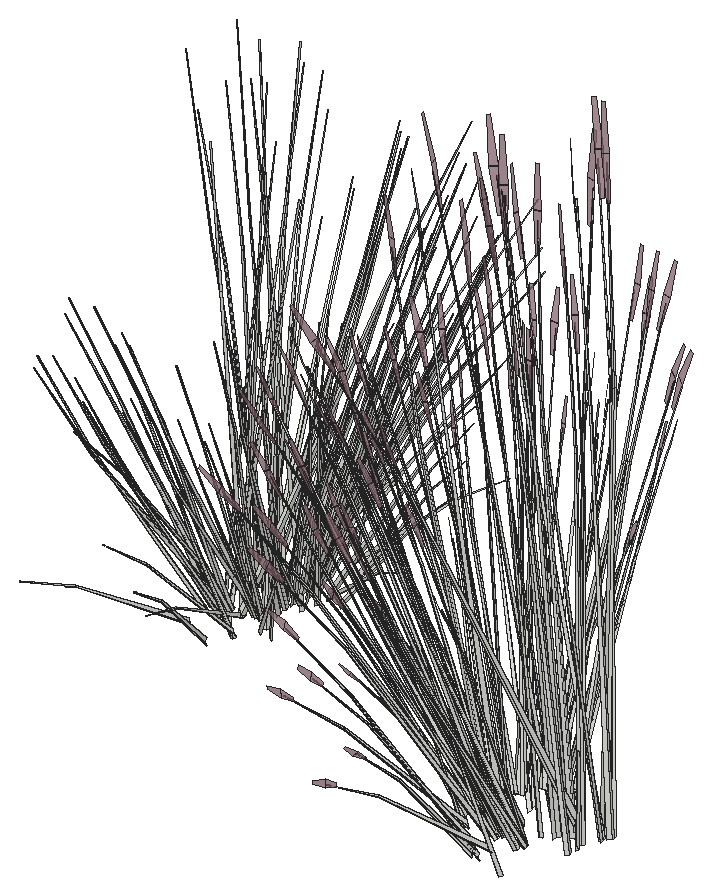
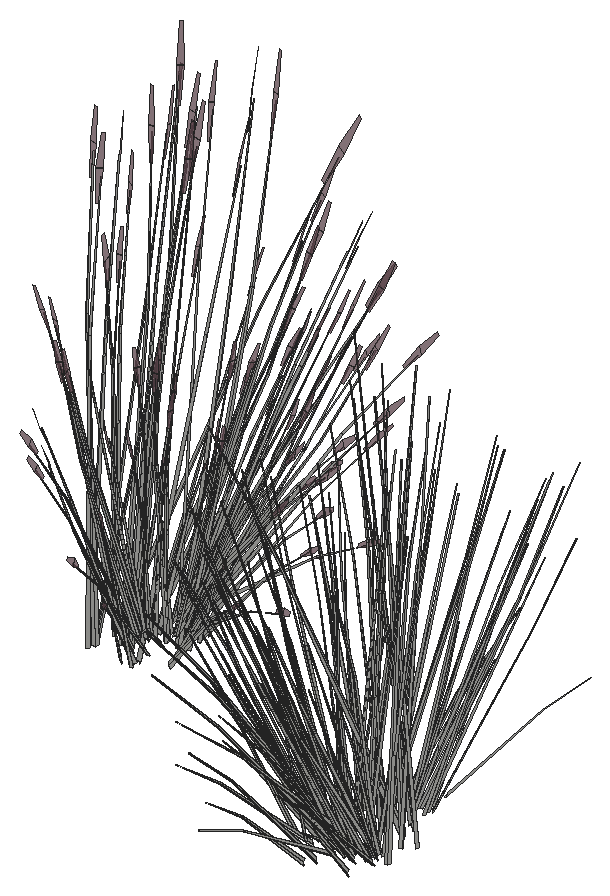
# SketchUp Ruby script. Lengths in inches.
U = 1.inch
M = Sketchup.active_model
def pt(a) = Geom::Point3d.new(a.map { |v| v * U })
def face(e, loops, mat)
  f = e.add_face(loops[0].map { |a| pt(a) })
  loops[1..].each { |l| e.add_face(l.map { |a| pt(a) }).erase! }
  f.material = f.back_material = mat if mat
  f
end
# faces: each face lists its corners as indices into pts; further lists are holes
def faces(e, pts, list, mat = nil) = list.each { |f| face(e, (f[0].is_a?(Array) ? f : [f]).map { |l| l.map { |i| pts[i] } }, mat) }
# xy, xz, yz: faces in a plane at the given z, y or x. An outline is a flat list of corners, or four numbers for a rectangle; further outlines are holes
def ring(l) = l.size == 4 ? [[l[0], l[1]], [l[2], l[1]], [l[2], l[3]], [l[0], l[3]]] : l.each_slice(2).to_a
def flat(e, list, mat, &to3) = list.each { |f| face(e, (f[0].is_a?(Array) ? f : [f]).map { |l| ring(l).map { |u, v| to3.(u, v) } }, mat) }
def xy(e, z, list, mat = nil) = flat(e, list, mat) { |x, y| [x, y, z] }
def xz(e, y, list, mat = nil) = flat(e, list, mat) { |x, z| [x, y, z] }
def yz(e, x, list, mat = nil) = flat(e, list, mat) { |y, z| [x, y, z] }
def lines(e, pts, list) = list.each { |a, b| e.add_line(pt(pts[a]), pt(pts[b])) }
# prism: a flat outline (further loops are holes) pulled along v
def prism(e, loops, v, mat = nil)
  f = face(e, loops, mat); d = Geom::Vector3d.new(v.map { |x| x * U })
  f.pushpull(f.normal.samedirection?(d) ? d.length : -d.length)
end
def box(e, o, s, mat = nil) = prism(e, [[o, [o[0] + s[0], o[1], o[2]], [o[0] + s[0], o[1] + s[1], o[2]], [o[0], o[1] + s[1], o[2]]]], [0, 0, s[2]], mat)
def at(x, y, z, deg = 0) = Geom::Transformation.translation(pt([x, y, z])) * Geom::Transformation.rotation(ORIGIN, Z_AXIS, deg.degrees)
def axes(o, x, y, z) = Geom::Transformation.new([*x, 0, *y, 0, *z, 0, *pt(o).to_a, 1])
def part(name) = M.definitions.add(name)
# library, detail: a bought-in or finely detailed component or shape, given as its bounding box
def library(name, o, s) = part(name).tap { |d| box(d.entities, o, s) }
def detail(e, o, s) = box(e.add_group.entities, o, s)
def put(e, d, t, mat = nil) = e.add_instance(d, t).tap { |i| i.material = mat if mat }
def group(e, t, mat = nil) = e.add_group.tap { |g| g.transformation = t; g.material = mat if mat }.entities
root = M.entities
M.materials.add("LightPink_Translucent").color = [144, 107, 117]
M.materials["LightPink_Translucent"].alpha = 0.75
c1 = part("blade")
p = [[2.15,0.21,22],[0,0.17,0],[0.09,0.45,0],[2.18,0.31,22],[2.29,0.31,22],[0.38,0.45,0],
  [2.48,0.24,33],[2.49,0.24,33],[2.48,0.22,33]]
faces(c1.entities,p,[[0,1,2,3],[4,5,2,3],[6,3,4,7],[8,0,3,6]])
c2 = part("blade with seeds\#1")
put(c2.entities,c1,at(0,0,0))
c3 = part("seeds")
p = [[0.3,-0.1,1.38],[-0.01,-0.03,1.59],[-0.01,-0.03,0.03],[0.14,-0.07,-0.07],[0.29,-0.03,3],[0.15,0.01,3.11]]
faces(c3.entities,p,[[0,1,2,3],[1,0,4,5]],"LightPink_Translucent")
c4 = part("blade with seeds")
put(c4.entities,c1,at(0,0,0))
put(c4.entities,c3,axes([2.4,0.25,30.99],[1.5799,-0.05474,1.17369],[-0.12525,1.92788,0.29478],[-0.07173,-0.02425,1.56792]))
put(root,c2,axes([216.32,38.09,16.14],[-0.56782,-0.84974,0.42031],[0.60301,-0.73285,0.34656],[-0.10474,0.39867,0.86972]))
put(root,c2,axes([220.11,33.5,14.76],[0.31026,-0.88918,1.18253],[0.6684,0.87109,0.46763],[-0.39615,0.39018,0.99135]))
put(root,c2,axes([216.32,37.7,15.86],[-0.58508,-0.05181,0.05027],[0.01604,-0.78236,0.39574],[-0.06122,0.29969,0.60345]))
put(root,c2,axes([216.5,38,15.7],[-0.48173,0.58546,-0.27686],[-0.45602,-0.6685,0.35743],[-0.06938,0.33965,0.68391]))
put(root,c2,axes([217.37,29.3,15.7],[-0.10996,-0.89566,-0.27686],[0.6286,-0.2365,0.35743],[-0.16884,-0.25667,0.68391]))
put(root,c2,axes([217.74,30.03,16.11],[0.10996,0.89566,0.27686],[-0.6286,0.2365,-0.35743],[-0.16884,-0.25667,0.68391]))
put(root,c2,axes([216.83,37.38,16.06],[-0.01853,1.02857,-0.55542],[-0.78011,-0.06908,0.06703],[-0.08233,0.43575,0.78569]))
put(root,c2,axes([217.5,29.41,15.86],[0.70813,-0.25519,0.37528],[0.1229,1.00103,0.30943],[-0.16654,-0.29502,0.77654]))
put(root,c2,axes([217.64,29.22,15.86],[0.32359,-0.70638,0.05027],[0.4608,0.41126,0.39574],[-0.14898,-0.22647,0.60345]))
put(root,c2,axes([218.36,26.72,15.85],[-0.1172,-0.14278,1.36768],[-0.7189,0.18276,-0.2163],[-0.1363,-0.35826,0.10969]))
put(root,c2,axes([215.55,38.78,15.84],[0.07678,-0.07628,1.38675],[0.69023,0.36774,-0.13103],[0.00499,0.37243,0.24541]))
put(root,c2,axes([216.98,37.73,15.82],[0.50967,0.74714,-0.39948],[-0.5384,0.65433,-0.30943],[-0.07755,0.37961,0.76437]))
put(root,c2,axes([216.76,37.17,16.11],[0.48173,-0.58546,0.27686],[0.45602,0.6685,-0.35743],[-0.06938,0.33965,0.68391]))
put(root,c2,axes([218.625,34.39,14.0625],[0.37292,-1.15935,0.18813],[0.77487,0.55796,0.39091],[-0.17862,0,1.25509]))
put(root,c2,axes([216.45,37.33,16.1],[0.78248,0.05509,-0.09507],[-0.02139,1.04315,-0.52766],[-0.05435,0.40176,0.80177]))
put(root,c2,axes([217.66,39.41,14.32],[-0.05506,-0.65692,0.89796],[0.4851,0.4167,0.65976],[-0.07277,0.32462,0.19778]))
put(root,c2,axes([218.11,34.77,14.29],[0.0475,1.11735,0.34976],[-0.78843,0.10105,-0.16833],[-0.07991,-0.20003,1.12298]))
put(root,c2,axes([219.45,29.53,16.1],[-0.69671,0.51771,-0.09507],[-0.34238,-0.91885,-0.52766],[-0.09192,-0.38721,0.80177]))
put(root,c2,axes([217.53,38.66,15.19],[-0.01743,-0.42679,1.33979],[0.75527,0.28313,0.10833],[-0.04672,0.60821,0.57275]))
put(root,c2,axes([218.85,29.57,15.82],[-0.69988,-0.27875,-0.39948],[0.23989,-0.95572,-0.30943],[-0.06417,-0.38479,0.76437]))
put(root,c2,axes([219.07,35.03,14.29],[0.6933,0.49923,0.34976],[-0.33366,1.03732,-0.16833],[-0.15982,0,1.12298]))
put(root,c2,axes([216.75,35.29,14.1],[0.76467,0.29724,0.13792],[-0.21639,1.08771,0.2743],[-0.00372,-0.1879,1.25403]))
put(root,c2,axes([219.11,29.75,16.06],[-0.33981,-0.90415,-0.55542],[0.69949,-0.50388,0.06703],[-0.07946,-0.43686,0.78569]))
put(root,c2,axes([219.24,29.89,16.11],[-0.21464,0.85512,0.27686],[-0.6262,-0.24941,-0.35743],[-0.05742,-0.34428,0.68391]))
put(root,c2,axes([218.1,38.84,15.86],[-0.70155,-0.2907,0.37528],[0.23989,-0.95572,0.30943],[0.04216,0.37584,0.77654]))
put(root,c2,axes([217.91,38.91,15.86],[-0.52462,0.37791,0.05027],[-0.25678,-0.68914,0.39574],[0.05066,0.30378,0.60345]))
put(root,c2,axes([217.78,33.43,14.29],[-0.64581,0.61812,0.34976],[-0.45477,-0.93627,-0.16833],[0.07991,-0.20003,1.12298]))
put(root,c2,axes([216.8,32,14.1],[0.20421,1.10567,0.13792],[-0.75999,0.27302,0.2743],[0.11073,-0.09861,1.25403]))
put(root,c2,axes([218.18,39.04,15.7],[-0.21464,0.85512,-0.27686],[-0.6262,-0.24941,0.35743],[0.05742,0.34428,0.68391]))
put(root,c2,axes([219.17,28.99,15.7],[0.21464,-0.85512,-0.27686],[0.6262,0.24941,0.35743],[-0.05742,-0.34428,0.68391]))
put(root,c2,axes([220.7,35.39,14.1],[-0.20421,-1.10567,0.13792],[0.75999,-0.27302,0.2743],[-0.11073,0.09861,1.25403]))
put(root,c2,axes([218.4,31.32,15.19],[0.01743,0.42679,1.33979],[-0.75527,-0.28313,0.10833],[0.04672,-0.60821,0.57275]))
put(root,c2,axes([219.4375,29.11,15.86],[0.52462,-0.37791,0.05027],[0.25678,0.68914,0.39574],[-0.05066,-0.30378,0.60345]))
put(root,c2,axes([219.25,29.18,15.86],[0.70155,0.2907,0.37528],[-0.23989,0.95572,0.30943],[-0.04216,-0.37584,0.77654]))
put(root,c2,axes([218.11,38.14,16.11],[0.21464,-0.85512,0.27686],[0.6262,0.24941,-0.35743],[0.05742,0.34428,0.68391]))
put(root,c2,axes([218.79,30.41,14.1],[-0.56045,0.80843,0.13792],[-0.5436,-0.81469,0.2743],[0.11446,0.08929,1.25403]))
put(root,c2,axes([218.07,36.43,14.77],[-0.1113,-0.29248,1.38425],[0.77713,-0.10086,0.10833],[0.10312,0.63351,0.49474]))
put(root,c2,axes([219.3,27.17,14.32],[0.12702,0.63574,0.89796],[-0.52496,-0.29925,0.65976],[0.03592,-0.33726,0.19778]))
put(root,c2,axes([220.74,32.1,14.1],[-0.76467,-0.29724,0.13792],[0.21639,-1.08771,0.2743],[0.00372,0.1879,1.25403]))
put(root,c2,axes([218.42,32.36,14.29],[-0.6933,-0.49923,0.34976],[0.33366,-1.03732,-0.16833],[0.15982,0,1.12298]))
put(root,c2,axes([218.5,38.45,15.82],[0.69988,0.27875,-0.39948],[-0.23989,0.95572,-0.30943],[0.06417,0.38479,0.76437]))
put(root,c2,axes([217.9,38.5,16.1],[0.69671,-0.51771,-0.09507],[0.34238,0.91885,-0.52766],[0.09192,0.38721,0.80177]))
put(root,c2,axes([221.52,27.47,15.84],[-0.06736,0.09304,1.38675],[-0.72203,-0.20352,-0.13103],[-0.04613,-0.36649,0.24541]))
put(root,c2,axes([218.59,39.58,15.85],[0.0999,0.16803,1.36768],[0.72987,-0.01429,-0.2163],[0.09492,0.38514,0.10969]))
put(root,c2,axes([220.92,28.28,15.23],[-0.64678,0.19693,-0.0273],[-0.14869,-0.93082,-0.12377],[0.041,-0.19438,0.40823]))
put(root,c2,axes([220.9,30.6875,16.1],[-0.78248,-0.05509,-0.09507],[0.02139,-1.04315,-0.52766],[0.05435,-0.40176,0.80177]))
put(root,c2,axes([219.39,32.625,14.29],[-0.0475,-1.11735,0.34976],[0.78843,-0.10105,-0.16833],[0.07991,0.20003,1.12298]))
put(root,c2,axes([220.59,30.85,16.11],[-0.48173,0.58546,0.27686],[-0.45602,-0.6685,-0.35743],[0.06938,-0.33965,0.68391]))
put(root,c2,axes([220.43,29.78,15.85],[-0.01301,-0.22073,1.36768],[-0.59776,-0.60543,-0.2163],[0.0789,-0.39262,0.10969]))
put(root,c2,axes([219.71,38.81,15.86],[-0.32359,0.70638,0.05027],[-0.4608,-0.41126,0.39574],[0.14898,0.22647,0.60345]))
put(root,c2,axes([219.85,38.61,15.86],[-0.70813,0.25519,0.37528],[-0.1229,-1.00103,0.30943],[0.16654,0.29502,0.77654]))
put(root,c2,axes([218.86,38.48,15.19],[-0.16275,-0.35702,1.33979],[0.75203,-0.30057,0.10833],[0.16997,0.56048,0.57275]))
put(root,c2,axes([220.52,30.64,16.06],[0.01853,-1.02857,-0.55542],[0.78011,0.06908,0.06703],[0.08233,-0.43575,0.78569]))
put(root,c2,axes([219.61,37.99,16.11],[-0.10996,-0.89566,0.27686],[0.6286,-0.2365,-0.35743],[0.16884,0.25667,0.68391]))
put(root,c2,axes([219.33,41.44,15.84],[0.02064,-0.13132,1.38675],[0.67982,-0.40623,-0.13103],[0.17843,0.26881,0.24541]))
put(root,c2,axes([219.98,38.72,15.7],[0.10996,0.89566,-0.27686],[-0.6286,0.2365,0.35743],[0.16884,0.25667,0.68391]))
put(root,c2,axes([220.85,30.02,15.7],[0.48173,-0.58546,-0.27686],[0.45602,0.6685,0.35743],[0.06938,-0.33965,0.68391]))
put(root,c2,axes([221.03,30.32,15.86],[0.58508,0.05181,0.05027],[-0.01604,0.78236,0.39574],[0.06122,-0.29969,0.60345]))
put(root,c2,axes([220.84,30.25,15.86],[0.50698,0.7587,0.37528],[-0.5384,0.65433,0.30943],[0.09352,-0.35595,0.77654]))
put(root,c2,axes([221.49,40.34,14.32],[-0.34872,-0.42882,0.89796],[0.55204,-0.16921,0.65976],[0.09885,0.30989,0.19778]))
put(root,c2,axes([217.87,32.05,15.66],[-0.39977,0.88912,1.08107],[-0.62243,-0.93883,0.46645],[0.3751,-0.28686,1.04495]))
put(root,c2,axes([219.61,32.12,15.19],[-0.13256,0.3822,1.33979],[-0.55613,-0.79096,0.10833],[0.25088,-0.49297,0.57275]))
put(root,c2,axes([221.39,40.03,16.58],[0.20538,-0.90798,-0.05072],[0.63212,0.2793,-0.22997],[0.09598,0.14851,0.75852]))
put(root,c2,axes([221.43,32.66,16.11],[-0.61974,0.15892,0.27686],[-0.16365,-0.90846,-0.35743],[0.1776,-0.24401,0.68391]))
put(root,c2,axes([219.55,38.46,16.1],[0.42425,-0.9518,-0.09507],[0.6144,0.54834,-0.52766],[0.21357,0.26891,0.80177]))
put(root,c2,axes([221.12,30.71,14.32],[-0.22123,0.57934,0.89796],[-0.22479,-0.74807,0.65976],[0.19041,-0.20177,0.19778]))
put(root,c2,axes([219.36,37.18,15.19],[-0.23641,-0.257,1.33979],[0.63812,-0.64891,0.10833],[0.2906,0.44508,0.57275]))
put(root,c2,axes([220.05,37.99,15.82],[0.70255,-0.26433,-0.39948],[0.1229,1.00103,-0.30943],[0.1887,0.28686,0.76437]))
put(root,c2,axes([221.75,32.74,16.1],[-0.65859,-0.61314,-0.09507],[0.37942,-0.88794,-0.52766],[0.18607,-0.30866,0.80177]))
put(root,c2,axes([218.63,32.12,14.38],[-0.72443,0.02811,1.10444],[0.18779,-1.27212,0.46763],[0.3964,0.30088,1.0425]))
put(root,c2,axes([220.86,36.78,16.11],[-0.4051,-0.6962,0.27686],[0.46256,-0.65905,-0.35743],[0.23502,0.10028,0.68391]))
put(root,c2,axes([221.23,37.42,15.86],[-0.03585,0.84557,0.05027],[-0.54135,-0.02318,0.39574],[0.20737,0.08848,0.60345]))
put(root,c2,axes([222.3,33.55,15.84],[-0.09315,-0.00304,1.38675],[-0.41098,-0.88177,-0.13103],[0.14669,-0.30629,0.24541]))
put(root,c2,axes([221.28,37.15,15.86],[-0.52497,0.7327,0.37528],[-0.45276,-0.77811,0.30943],[0.2463,0.13515,0.77654]))
put(root,c2,axes([221.42,32.02,15.82],[-0.1829,-1.01534,-0.39948],[0.69265,-0.17761,-0.30943],[0.19849,-0.27272,0.76437]))
put(root,c2,axes([221.53,34.83,16.11],[-0.59169,-0.3102,0.27686],[0.17258,-0.905,-0.35743],[0.23822,-0.08298,0.68391]))
put(root,c2,axes([222.125,30.62,14.25],[-0.02413,0.65983,0.82134],[-0.51251,-0.43575,0.45348],[0.18208,-0.26066,0.64427]))
put(root,c2,axes([221.99,32.52,15.86],[0.48877,0.46765,0.05027],[-0.28456,0.66596,0.39574],[0.1567,-0.2153,0.60345]))
put(root,c2,axes([221.86,32.32,15.86],[0.17657,1.0234,0.37528],[-0.69265,0.17761,0.30943],[0.20414,-0.24069,0.77654]))
put(root,c2,axes([219.95,37.37,15.19],[-0.26446,-0.19158,1.33979],[0.54729,-0.80372,0.10833],[0.3411,0.36257,0.57275]))
put(root,c2,axes([223.64,33.61,16.58],[-0.4414,-0.71104,-0.05072],[0.48343,-0.65151,-0.22997],[0.13698,-0.04587,0.75852]))
put(root,c2,axes([221.4375,37.15,15.7],[0.4051,0.6962,-0.27686],[-0.46256,0.65905,0.35743],[0.23502,0.10028,0.68391]))
put(root,c2,axes([222.06,35.11,15.86],[0.26149,0.75819,0.05027],[-0.47684,0.37111,0.39574],[0.2102,-0.07322,0.60345]))
put(root,c2,axes([221.32,39.55,15.85],[0.15226,0.02558,1.36768],[0.52969,-0.72584,-0.2163],[0.25048,0.19002,0.10969]))
put(root,c2,axes([220.97,37.23,16.38],[0.03812,-1.13085,-0.10552],[0.7218,0.03091,-0.5857],[0.27799,0.07855,0.88996]))
put(root,c2,axes([222.01,34.84,16.12],[-0.20115,1.01389,0.41656],[-0.6613,-0.3467,0.34347],[0.26006,-0.06093,0.86196]))
put(root,c2,axes([221.78,35.14,16.1],[-0.35822,-1.00689,-0.09507],[0.63579,-0.49481,-0.52766],[0.26792,-0.13285,0.80177]))
put(root,c2,axes([223.01,36.7,14.32],[-0.4575,0.02663,0.89796],[0.32631,-0.6654,0.65976],[0.21806,0.13086,0.19778]))
put(root,c2,axes([221.25,36.46,16.07],[0.51698,-0.73658,-0.44342],[0.45276,0.77811,-0.34347],[0.26267,0.11207,0.84845]))
put(root,c2,axes([220.38,33.7,15.19],[-0.24703,0.23521,1.33979],[-0.20797,-1.08685,0.10833],[0.38782,-0.24564,0.57275]))
put(root,c2,axes([221.75,34.27,15.82],[0.19288,-1.01147,-0.39948],[0.6613,0.3467,-0.30943],[0.26625,-0.09275,0.76437]))
put(root,c2,axes([222.15,34.73,15.7],[0.59169,0.3102,-0.27686],[-0.17258,0.905,0.35743],[0.23822,-0.08298,0.68391]))
put(root,c2,axes([221.01,36.68,16.33],[0.71171,0.02677,-0.61651],[-0.0478,1.12742,0.0744],[0.30151,0.11898,0.87212]))
put(root,c2,axes([220.5,35.62,15.19],[-0.29531,0.02518,1.33979],[0.19591,-1.09152,0.10833],[0.42084,0.06751,0.57275]))
put(root,c2,axes([222.88,39.63,15.84],[-0.04645,-0.11673,1.38675],[0.30899,-0.96483,-0.13103],[0.25727,0.02267,0.24541]))
put(root,c2,axes([221.62,34.64,16.06],[0.62562,-0.4911,-0.55542],[0.34866,1.01092,0.06703],[0.30228,-0.11484,0.78569]))
put(root,c2,axes([223.2,35.375,15.85],[0.1239,-0.13043,1.36768],[0.04868,-1.05257,-0.2163],[0.27325,-0.10585,0.10969]))
put(root,c2,axes([222.01,37.0625,14.79],[-0.3972,-0.02261,1.20664],[0.2098,-1.0168,0.16675],[0.42332,0.0881,0.56978]))
put(root,c4,axes([250.125,18.36,15.95],[0.4003,-0.02088,1.4862],[-0.26555,0.90478,0.12017],[-0.57046,-0.05596,0.63534]))
put(root,c4,axes([250.29,19.95,15.95],[0.33486,-0.19497,1.4862],[0.28191,0.90091,0.12017],[-0.52569,0.20361,0.63534]))
put(root,c4,axes([249.25,21.49,14.84],[0.33539,0.07567,1.24013],[0.21617,0.77287,-0.2667],[-0.45558,0.14467,0.53022]))
put(root,c4,axes([252.22,19.01,15.49],[0.27432,-0.13334,1.53553],[0.0946,0.93098,0.12017],[-0.59418,0.12354,0.54881]))
put(root,c4,axes([249.27,19.64,16.68],[-0.1576,0.11967,1.51715],[0.01341,0.87436,-0.23994],[-0.36123,0.11371,0.12168]))
put(root,c4,axes([251.32,17.52,16.91],[-0.96472,-0.02219,-0.61612],[0.06479,-0.93454,0.07435],[-0.4087,-0.09862,0.87156]))
put(root,c4,axes([250.54,17.75,14.84],[0.18842,0.25662,1.24013],[-0.43418,0.69755,-0.2667],[-0.44582,-0.16673,0.53022]))
put(root,c4,axes([249.77,19.14,16.52],[-0.80204,-0.25713,-0.30711],[0.23393,-0.75017,0.39649],[-0.32291,0.06879,0.75865]))
put(root,c4,axes([250.88,16.91,15.95],[0.35848,0.15881,1.4862],[-0.74185,0.66622,0.12017],[-0.46237,-0.30054,0.63534]))
put(root,c4,axes([247.52,20.52,16.68],[0.12316,0.02472,1.5383],[0.38101,0.8144,-0.14535],[-0.25212,0.21376,0.27223]))
put(root,c4,axes([250.32,19.52,16.65],[-0.26145,0.83843,-0.44314],[-0.89639,-0.28738,-0.34325],[-0.3609,0.07688,0.8479]))
put(root,c4,axes([251,17.71,16.65],[-0.70076,0.61057,-0.44314],[-0.61371,-0.64499,-0.34325],[-0.35604,-0.0929,0.8479]))
put(root,c4,axes([250.01,16,16.68],[0.07154,0.09199,1.5383],[-0.34491,0.82687,-0.14535],[-0.34931,0.00598,0.27223]))
put(root,c4,axes([248.55,23.11,14.99],[0.4022,-0.41775,0.99609],[0.1587,0.66133,0.73186],[-0.29065,0.11842,0.2194]))
put(root,c4,axes([250.8125,15.45,16.68],[-0.20765,-0.00651,1.51715],[-0.66108,0.65062,-0.23994],[-0.35273,-0.13294,0.12168]))
put(root,c4,axes([249.96,19.04,16.7],[0.27266,-0.84043,0.41629],[0.89639,0.28738,0.34325],[-0.35251,0.05051,0.8614]))
put(root,c4,axes([250.28,18.8,16.96],[0.48557,0.83463,-0.10546],[-0.86181,0.41016,-0.58532],[-0.36317,0.11012,0.88939]))
put(root,c4,axes([251.37,17.07,16.96],[-0.05167,0.93738,-0.10546],[-0.97839,-0.02562,-0.58532],[-0.37682,-0.06511,0.88939]))
put(root,c4,axes([250.74,17.13,16.52],[-0.54911,-0.5771,-0.30711],[0.627,-0.5463,0.39649],[-0.31857,-0.08312,0.75865]))
put(root,c4,axes([249.89,18.82,16.69],[-0.35445,-0.62848,0.05576],[0.64636,-0.30762,0.43899],[-0.28492,0.06069,0.6694]))
put(root,c4,axes([251.52,20.56,15.95],[0.24104,-0.28321,1.4862],[0.60863,0.76445,0.12017],[-0.41745,0.34813,0.63534]))
put(root,c4,axes([250.07,21.3,16.52],[-0.84006,0.13173,-0.30711],[-0.22182,-0.75304,0.39649],[-0.24073,0.20226,0.75865]))
put(root,c4,axes([249.42,18.52,14.99],[0.61613,-0.06596,0.99609],[-0.39083,0.58114,0.73186],[-0.30447,-0.08718,0.2194]))
put(root,c4,axes([250.18,21.14,16.7],[-0.23935,-0.84832,0.41629],[0.93889,-0.14723,0.34325],[-0.27671,0.19951,0.8614]))
put(root,c4,axes([250.66,16.92,17.01],[0.79699,-0.68023,0.46624],[0.68736,0.72239,0.38444],[-0.37392,-0.12548,0.96477]))
put(root,c4,axes([249.99,20.97,16.69],[-0.66253,-0.38765,0.05576],[0.38573,-0.55202,0.43899],[-0.21241,0.17847,0.6694]))
put(root,c4,axes([251.34,21.26,15.95],[0.17969,-0.31682,1.4862],[0.75383,0.65564,0.12017],[-0.34007,0.40863,0.63534]))
put(root,c4,axes([250.62,19.05,16.97],[0.80204,0.25713,0.30711],[-0.23393,0.75017,-0.39649],[-0.32291,0.06879,0.75865]))
put(root,c4,axes([250.76,21.39,16.65],[0.24792,0.84163,-0.44314],[-0.93889,0.14723,-0.34325],[-0.26906,0.22606,0.8479]))
put(root,c4,axes([251.02,16.91,16.69],[0.0486,-0.70091,0.05576],[0.7338,0.01922,0.43899],[-0.28109,-0.07334,0.6694]))
put(root,c4,axes([249.29,22.9,16.68],[-0.02399,0.1824,1.51715],[0.68078,0.63455,-0.23994],[-0.17822,0.30007,0.12168]))
put(root,c4,axes([253.28,15.7,17.3],[-0.64409,0.88364,-0.11811],[-0.93276,-0.50908,-0.65556],[-0.32423,-0.24965,0.99612]))
put(root,c4,axes([251.52,17.4375,16.97],[0.54911,0.5771,0.30711],[-0.627,0.5463,-0.39649],[-0.31857,-0.08312,0.75865]))
put(root,c4,axes([253,16.42,16.91],[-0.82291,-0.44552,-0.61612],[0.58483,-0.7807,0.07435],[-0.29815,-0.26601,0.87156]))
put(root,c4,axes([252.62,16.44,16.65],[-0.95231,0.21911,-0.44314],[-0.16659,-0.82977,-0.34325],[-0.25579,-0.23779,0.8479]))
put(root,c4,axes([250.32,20.79,16.96],[0.89271,0.50824,-0.10546],[-0.5143,0.73603,-0.58532],[-0.25221,0.25585,0.88939]))
put(root,c4,axes([252.33,23.11,14.65],[-0.60338,0.92363,0],[-1.00947,-0.51509,-0.44755],[-0.22991,-0.11731,1.41973]))
put(root,c4,axes([248.84,22.99,17.49],[0.85161,0.24604,-0.05626],[-0.26197,0.75726,-0.2551],[-0.13929,0.11498,0.84141]))
put(root,c4,axes([250.75,20.85,16.97],[0.84006,-0.13173,0.30711],[0.22182,0.75304,-0.39649],[-0.24073,0.20226,0.75865]))
put(root,c4,axes([251.23,24.44,14.84],[0.30454,-0.14541,1.24013],[0.75191,0.43843,-0.2667],[-0.2238,0.37937,0.53022]))
put(root,c4,axes([250.8,16.15,14.4375],[-0.27839,0.75264,-0.03376],[-0.85684,-0.23152,-0.15306],[-0.1301,-0.1231,0.50485]))
put(root,c4,axes([253.03,13.6,16.68],[-0.018,0.11048,1.5383],[-0.88797,0.40096,-0.14535],[-0.2613,-0.20496,0.27223]))
put(root,c4,axes([252.08,15.2,14.84],[-0.05844,0.30153,1.24013],[-0.85435,0.25241,-0.2667],[-0.1997,-0.38973,0.53022]))
put(root,c4,axes([252.36,15.98,15.95],[0.2206,0.29594,1.4862],[-1.01938,0.24915,0.12017],[-0.23039,-0.4646,0.63534]))
put(root,c4,axes([251.55,22.85,16.7],[-0.68722,-0.6289,0.41629],[0.72981,-0.54239,0.34325],[-0.12676,0.29506,0.8614]))
put(root,c4,axes([252.72,15.83,16.52],[-0.14905,-0.74243,-0.30711],[0.85206,-0.19604,0.39649],[-0.22886,-0.21276,0.75865]))
put(root,c4,axes([250.34,19.59,14.65],[-1.20676,0,0],[0,-1.03017,-0.44755],[0,-0.23463,1.41973]))
put(root,c4,axes([251.29,22.8,16.69],[-0.79307,-0.04295,0.05576],[0.02174,-0.64852,0.43899],[-0.08299,0.24842,0.6694]))
put(root,c4,axes([251.54,23.04,16.52],[-0.65298,0.48529,-0.30711],[-0.61814,-0.55413,0.39649],[-0.09405,0.28154,0.75865]))
put(root,c4,axes([253.22,16.43,16.97],[0.14905,0.74243,0.30711],[-0.85206,0.19604,-0.39649],[-0.22886,-0.21276,0.75865]))
put(root,c4,axes([249.22,24.77,16.68],[0.10948,-0.05565,1.5383],[0.90493,0.37016,-0.14535],[-0.02127,0.3082,0.27223]))
put(root,c4,axes([251.27,19.32,14.61],[-0.89767,0.77493,0.26672],[-0.89822,-0.76678,-0.31646],[-0.03135,-0.22007,1.42991]))
put(root,c4,axes([254.97,21.46,15.48],[0.83398,0.37168,1.31176],[-0.81701,0.80073,0.51873],[-0.36596,-0.47458,1.09968]))
put(root,c4,axes([251.79,14.72,14.99],[0.50342,0.32081,0.99609],[-0.73316,0.19284,0.73186],[-0.15687,-0.24655,0.2194]))
put(root,c4,axes([251.98,22.53,17.22],[-0.02511,0.8526,-0.68389],[-1.05743,-0.05726,0.08253],[-0.11159,0.3612,0.96743]))
put(root,c4,axes([251.96,24.93,14.99],[-0.02498,-0.54806,0.99609],[0.6241,0.3909,0.73186],[-0.12274,0.26123,0.2194]))
put(root,c4,axes([252.84,15.56,17.01],[1.07506,-0.23691,0.46624],[0.18658,0.92935,0.38444],[-0.25284,-0.2739,0.96477]))
put(root,c4,axes([253.08,15.76,16.69],[0.43862,-0.58553,0.05576],[0.62461,0.3409,0.43899],[-0.20194,-0.18773,0.6694]))
put(root,c4,axes([252.85,22.62,14.74],[0.90321,0.46087,0.43058],[-0.53987,0.8264,0],[-0.20571,-0.10497,1.3659]))
put(root,c4,axes([251.625,23.73,15.51],[0.0212,-0.47583,1.33851],[0.95368,0.25133,0.18497],[-0.08263,0.50712,0.63204]))
put(root,c4,axes([254.15,21.1875,14.86],[-0.18618,0.8226,0.12557],[-0.90961,-0.14279,-0.35857],[-0.16554,-0.08447,1.09915]))
put(root,c4,axes([254.04,14.02,16.68],[-0.14761,-0.12923,1.51715],[-0.98508,0.08193,-0.23994],[-0.15722,-0.30911,0.12168]))
put(root,c4,axes([251.07,19.74,14.74],[0,0.92173,0.43058],[-1.07973,0,0],[0,-0.20993,1.3659]))
put(root,c4,axes([256.02,23.23,14.49],[-0.59586,-0.92686,-0.04459],[1.00947,-0.51509,0.44755],[-0.24875,0.08824,1.41903]))
put(root,c4,axes([252.19,22.8125,16.93],[0.69086,0.61932,-0.49188],[-0.72981,0.54239,-0.381],[-0.10512,0.31467,0.94117]))
put(root,c4,axes([251.89,22.36,16.97],[0.65298,-0.48529,0.30711],[0.61814,0.55413,-0.39649],[-0.09405,0.28154,0.75865]))
put(root,c4,axes([256.26,19.68,15.06],[-0.02636,-0.86785,1.22513],[1.19315,0.22496,0.51873],[-0.2822,0.47488,1.15643]))
put(root,c4,axes([251.47,22.49,17.27],[1.06065,0.04567,-0.11706],[-0.02899,0.86469,-0.64971],[-0.07368,0.33302,0.98722]))
put(root,c4,axes([251.44,23.74,15.04],[0.87672,-0.16322,0.05643],[0.20155,0.65759,-0.74845],[-0.05558,0.33288,0.67088]))
put(root,c4,axes([255.54,16.02,16.96],[-0.94439,0.42914,-0.10546],[-0.46409,-0.76165,-0.58532],[-0.1246,-0.32096,0.88939]))
put(root,c4,axes([254.73,16.05,16.65],[-0.94868,-0.23106,-0.44314],[0.32517,-0.79222,-0.34325],[-0.08699,-0.31896,0.8479]))
put(root,c4,axes([252.98,21.93,15.95],[-0.02362,-0.35377,1.4862],[1.02376,0.23469,0.12017],[-0.06332,0.50416,0.63534]))
put(root,c4,axes([254.11,15.19,14.4375],[-0.6669,0.52879,-0.03376],[-0.61107,-0.57914,-0.15306],[-0.04302,-0.1641,0.50485]))
put(root,c4,axes([253.85,20.41,14.64],[1.21977,0.1942,0.39679],[-0.24824,1.0968,0.15571],[-0.17826,-0.10591,1.37763]))
put(root,c4,axes([253.53,20.21,14.95],[-0.46824,0.83055,0.38798],[-0.97292,-0.39972,-0.18672],[0,-0.19146,1.2457]))
put(root,c4,axes([255.08,16.21,16.91],[-0.46061,-0.74947,-0.61612],[0.94816,-0.41768,0.07435],[-0.10771,-0.36212,0.87156]))
put(root,c4,axes([253.19,22.16,14.74],[1.03704,-0.24464,0.153],[0.25607,0.91045,0.30427],[-0.09249,-0.13265,1.39107]))
put(root,c4,axes([254.53,22.3,14.5],[-0.97292,-0.41382,0],[0.46824,-0.85985,0],[0,0,1.41102]))
put(root,c4,axes([255.26,16.32,16.97],[-0.29095,0.70883,0.30711],[-0.84882,-0.20674,-0.39649],[-0.07783,-0.28538,0.75865]))
put(root,c4,axes([256.78,23.34,14.65],[0.60338,0.92363,0],[-1.00947,0.51509,-0.44755],[-0.22991,0.11731,1.41973]))
put(root,c4,axes([253.71,23.74,16.98],[-0.95095,-0.24097,0.46208],[0.32517,-0.79222,0.381],[0.05715,0.31154,0.95616]))
put(root,c4,axes([253.45,23.8,16.69],[-0.71112,0.31326,0.05576],[-0.34807,-0.57124,0.43899],[0.06868,0.25181,0.6694]))
put(root,c4,axes([256.28,22.21,14.74],[0.27879,-0.91605,0.153],[1.02019,0.25923,0.30427],[-0.17623,0.00446,1.39107]))
put(root,c4,axes([255.81,20.99,14.86],[0.71299,0.5538,0.12557],[-0.59472,0.6248,-0.35857],[-0.16554,0.08447,1.09915]))
put(root,c4,axes([255.55,20.31,14.58],[-0.89767,-0.79335,-0.05317],[0.89822,-0.79383,0],[-0.03135,-0.0277,1.52258]))
put(root,c4,axes([255.79,20.59,14.95],[1.04798,-0.0569,0.38798],[0.09477,0.94451,-0.18672],[-0.18761,0.09573,1.2457]))
put(root,c4,axes([256.04,22.76,14.61],[1.2082,0.29959,0.26672],[-0.30227,1.07087,-0.31646],[-0.19997,0.13403,1.42991]))
put(root,c4,axes([256.5625,22.7,14.74],[0.90321,-0.46087,0.43058],[0.53987,0.8264,0],[-0.20571,0.10497,1.3659]))
